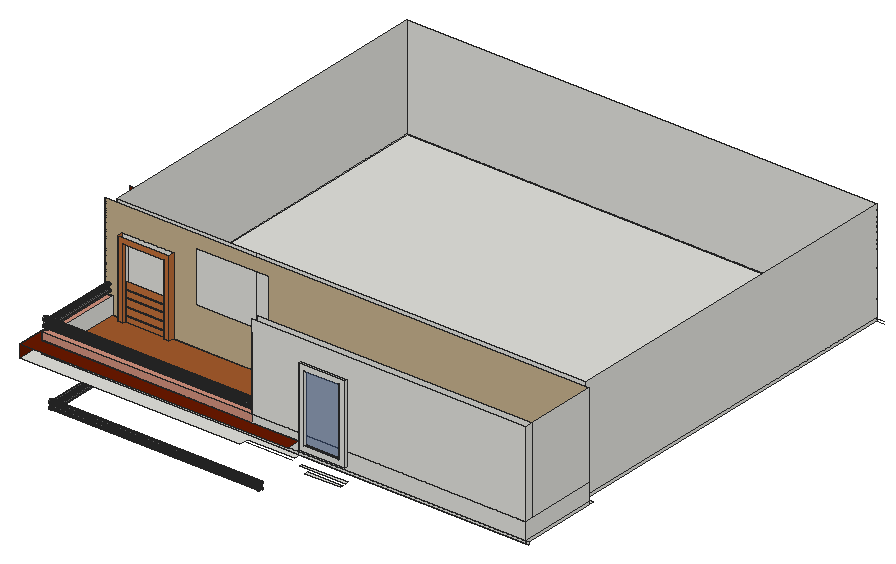
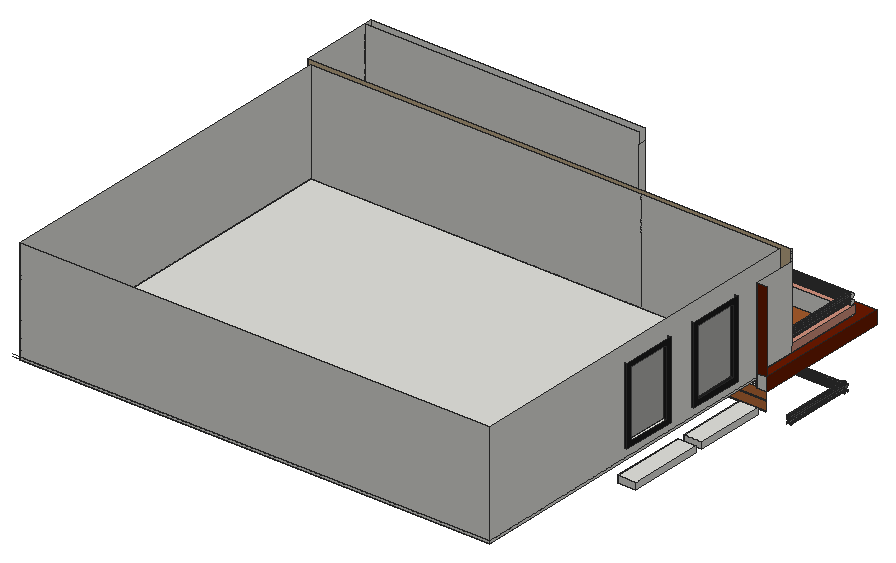
# SketchUp Ruby script. Lengths in inches.
U = 1.inch
M = Sketchup.active_model
def pt(a) = Geom::Point3d.new(a.map { |v| v * U })
def face(e, loops, mat)
  f = e.add_face(loops[0].map { |a| pt(a) })
  loops[1..].each { |l| e.add_face(l.map { |a| pt(a) }).erase! }
  f.material = f.back_material = mat if mat
  f
end
# faces: each face lists its corners as indices into pts; further lists are holes
def faces(e, pts, list, mat = nil) = list.each { |f| face(e, (f[0].is_a?(Array) ? f : [f]).map { |l| l.map { |i| pts[i] } }, mat) }
# xy, xz, yz: faces in a plane at the given z, y or x. An outline is a flat list of corners, or four numbers for a rectangle; further outlines are holes
def ring(l) = l.size == 4 ? [[l[0], l[1]], [l[2], l[1]], [l[2], l[3]], [l[0], l[3]]] : l.each_slice(2).to_a
def flat(e, list, mat, &to3) = list.each { |f| face(e, (f[0].is_a?(Array) ? f : [f]).map { |l| ring(l).map { |u, v| to3.(u, v) } }, mat) }
def xy(e, z, list, mat = nil) = flat(e, list, mat) { |x, y| [x, y, z] }
def xz(e, y, list, mat = nil) = flat(e, list, mat) { |x, z| [x, y, z] }
def yz(e, x, list, mat = nil) = flat(e, list, mat) { |y, z| [x, y, z] }
def lines(e, pts, list) = list.each { |a, b| e.add_line(pt(pts[a]), pt(pts[b])) }
# prism: a flat outline (further loops are holes) pulled along v
def prism(e, loops, v, mat = nil)
  f = face(e, loops, mat); d = Geom::Vector3d.new(v.map { |x| x * U })
  f.pushpull(f.normal.samedirection?(d) ? d.length : -d.length)
end
def box(e, o, s, mat = nil) = prism(e, [[o, [o[0] + s[0], o[1], o[2]], [o[0] + s[0], o[1] + s[1], o[2]], [o[0], o[1] + s[1], o[2]]]], [0, 0, s[2]], mat)
def at(x, y, z, deg = 0) = Geom::Transformation.translation(pt([x, y, z])) * Geom::Transformation.rotation(ORIGIN, Z_AXIS, deg.degrees)
def axes(o, x, y, z) = Geom::Transformation.new([*x, 0, *y, 0, *z, 0, *pt(o).to_a, 1])
def part(name) = M.definitions.add(name)
# library, detail: a bought-in or finely detailed component or shape, given as its bounding box
def library(name, o, s) = part(name).tap { |d| box(d.entities, o, s) }
def detail(e, o, s) = box(e.add_group.entities, o, s)
def put(e, d, t, mat = nil) = e.add_instance(d, t).tap { |i| i.material = mat if mat }
def group(e, t, mat = nil) = e.add_group.tap { |g| g.transformation = t; g.material = mat if mat }.entities
root = M.entities
M.materials.add("[0032_Moccasin]").color = [198, 177, 141]
M.materials.add("[0134_DimGray]").color = [105, 105, 105]
M.materials.add("[Color B02]").color = [209, 145, 125]
M.materials.add("[Color B07]").color = [107, 26, 0]
M.materials.add("[Color M08]").color = [30, 30, 30]
M.materials.add("[Translucent Glass Blue]").color = [61, 91, 145]
M.materials["[Translucent Glass Blue]"].alpha = 0.5
M.materials.add("[Translucent Glass Gray]").color = [128, 128, 128]
M.materials["[Translucent Glass Gray]"].alpha = 0.5
M.materials.add("[Wood Square Tile 01]").color = [164, 91, 44]
M.materials.add("[Wood Veneer 01]").color = [191, 111, 58]
xy(root,210,[[67.4,113.9375,115.4,116.9375],[67.4,116.9375,115.4,119.9375]])
xy(root,216,[[61.4,113.9375,121.4,119.9375]],"[Wood Veneer 01]")
xy(root,222.875,[[152.96,116.9375,192.8,119.9375],[195.8,116.9375,232.65,119.9375]],"[Color M08]")
xy(root,225.875,[[149.96,116.9375,235.65,119.9375]])
xy(root,228.99,[[31.875,209.04,34.875,261.16],[31.875,301.91,34.875,354.04]],"[Color M08]")
xy(root,234.99,[[13.875,196.1,13.875,278.07,34.875,278.07,34.875,267.16,31.875,267.16,31.875,203.04,34.875,203.04,34.875,196.1],[31.875,203.04,34.875,267.16],[13.875,286.99,13.875,375.6,34.875,375.6,34.875,360.04,31.875,360.04,31.875,295.91,34.875,295.91,34.875,286.99],[31.875,295.91,34.875,360.04]])
xy(root,235.15,[[352.1,17.9375,393.78,20.9375]])
xy(root,241.15,[[346.1,17.9375,399.78,20.9375]])
xy(root,242.93,[[13.875,196.1,34.875,278.07],[13.875,286.99,34.875,375.6]])
xy(root,244.83,[[23.625,9.86,23.625,170.67,34.875,170.67,34.875,119.9375,337.625,119.9375,337.625,20.9375,282.125,20.9375,282.125,9.86]])
xy(root,246,[[34.875,26.9375,282.125,37.04],[282.125,26.9375,337.625,37.04],[337.625,26.9375,604.125,44.9375],[34.875,37.04,34.875,119.9375,337.625,119.9375,337.625,44.9375,282.125,44.9375,282.125,37.04],[282.125,37.04,337.625,44.9375],
  [337.625,44.9375,604.125,119.9375],[207.54,119.9375,595.125,125.9375],[595.125,119.9375,603.5625,125.9375],[43.875,125.9375,595.125,552.98]])
xy(root,249,[[34.875,26.9375,34.875,119.9375,43.875,119.9375,43.875,35.9375,595.125,35.9375,595.125,119.9375,604.125,119.9375,604.125,26.9375],[55.4,113.9375,61.4,119.9375],[109.4,113.9375,115.4,119.9375],[61.4,116.9375,109.4,119.9375],[43.875,125.9375,595.125,552.98]])
xy(root,249,[[43.875,35.9375,595.125,35.9375,595.125,119.9375,115.4,119.9375,115.4,113.9375,109.4,113.9375,109.4,116.9375,61.4,116.9375,61.4,113.9375,55.4,113.9375,55.4,119.9375,43.875,119.9375]],"[Wood Square Tile 01]")
xy(root,257.08,[[344.26,17.9375,397.95,20.9375]])
xy(root,260.11,[[23.625,9.86,337.625,9.86,337.625,26.9375,34.875,26.9375,34.875,170.67,23.625,170.67]],"[Color B07]")
xy(root,263.08,[[350.26,17.9375,391.95,20.9375]])
xy(root,266.99,[[31.875,203.04,34.875,267.16],[31.875,301.48,34.875,365.6]],"[Color M08]")
xy(root,268.875,[[282.125,26.9375,604.125,35.9375],[595.125,35.9375,604.125,119.9375]])
xy(root,268.875,[[34.875,26.9375,282.125,26.9375,282.125,35.9375,43.875,35.9375,43.875,119.9375,34.875,119.9375]],"[Color B02]")
xy(root,272.99,[[31.875,307.48,34.875,359.6]])
xy(root,272.99,[[31.875,209.04,34.875,261.16]],"[Color M08]")
xz(root,17.9375,[[[344.26,257.08,397.95,348.9],[350.26,263.08,391.95,342.9]]])
xz(root,20.9375,[[[344.26,257.08,397.95,348.9],[350.26,263.08,391.95,342.9]]])
xz(root,20.9375,[[350.26,263.08,391.95,342.9]],"[Translucent Glass Blue]")
xz(root,26.9375,[[34.875,246,282.125,249],[282.125,246,337.625,249],[337.625,246,604.125,249],[604.125,246,607.125,249],[34.875,249,282.125,260.11],
  [282.125,249,337.625,260.11],[337.625,249,337.625,260.11,282.125,260.11,282.125,268.875,604.125,268.875,604.125,249],[282.125,268.875,604.125,369]])
xz(root,26.9375,[[34.875,260.11,282.125,268.875]],"[Color B02]")
xz(root,29.17,[[39.53,271.5,40.08,271.57,40.59,271.78,41.03,272.12,41.37,272.5625,41.58,273.07,41.66,273.625,41.66,273.63,37.41,273.63,37.41,273.625,37.48,273.07,37.69,272.5625,38.03,272.12,38.47,271.78,38.98,271.57],[37.41,273.63,41.66,273.63,41.58,274.17,41.37,274.6875,41.24,274.86,37.82,274.86,37.69,274.6875,37.48,274.17],[37.82,274.86,41.24,274.86,41.03,275.125,40.59,275.46,40.08,275.68,39.53,275.75,38.98,275.68,38.47,275.46,38.03,275.125]])
xz(root,35.9375,[[43.875,249,282.125,268.875],[282.125,249,595.125,268.875],[282.125,268.875,604.125,369]])
xz(root,113.9375,[[55.4,249,61.4,249,61.4,333,109.4,333,109.4,249,115.4,249,115.4,339,55.4,339]],"[Wood Veneer 01]")
xz(root,116.9375,[[67.4,185.27,115.4,186.19],[67.4,196.84,115.4,197.75],[61.4,255.89,109.4,256.87],[61.4,264.83,109.4,265.81],[61.4,274.08,109.4,275.06],
  [61.4,283.33,109.4,284.31]])
xz(root,116.9375,[[67.4,186.19,115.4,196.84],[67.4,197.75,115.4,210],[61.4,249,109.4,255.89],[61.4,256.87,109.4,264.83],[61.4,265.81,109.4,274.08],
  [61.4,275.06,109.4,283.33],[61.4,284.31,109.4,292.58]],"[Wood Veneer 01]")
xz(root,119.9375,[[34.875,244.83,337.625,246],[34.875,246,43.875,249],[43.875,246,55.4,249],[55.4,246,115.4,249],[115.4,246,207.54,249],
  [207.54,246,595.125,249],[595.125,246,603.4375,249],[603.4375,246,603.5625,249],[603.5625,246,604.125,249],[34.875,249,35.6,268.875],
  [35.6,249,43.875,268.875],[55.4,249,55.4,339,115.4,339,115.4,249,109.4,249,109.4,333,61.4,333,61.4,249],[61.4,249,109.4,333],[595.125,249,603.4375,268.875],[603.4375,249,603.5625,268.875],
  [603.5625,249,604.125,268.875],[34.875,268.875,35.6,369]])
xz(root,119.9375,[[[43.875,249,55.4,249,55.4,339,115.4,339,115.4,249,595.125,249,595.125,268.875,604.125,268.875,604.125,369,35.6,369,35.6,268.875,43.875,268.875],[141.33,293.5,227.02,354.1875],[39.53,271.5,38.98,271.57,38.47,271.78,38.03,272.12,37.69,272.5625,37.48,273.07,37.41,273.625,37.48,274.17,37.69,274.6875,38.03,275.125,38.47,275.46,38.98,275.68,39.53,275.75,40.08,275.68,40.59,275.46,41.03,275.125,41.37,274.6875,41.58,274.17,41.66,273.625,41.58,273.07,41.37,272.5625,41.03,272.12,40.59,271.78,40.08,271.57]]],"[0032_Moccasin]")
xz(root,125.9375,[[43.875,246,207.54,249],[207.54,246,595.125,249],[43.875,249,207.54,369],[207.54,249,595.125,369]])
xz(root,170.67,[[23.625,244.83,34.875,260.11]])
xz(root,170.67,[[23.625,260.11,34.875,355.125]],"[Color B07]")
xz(root,196.1,[[13.875,234.99,34.875,242.93]])
xz(root,203.04,[[31.875,266.99,34.875,357.43]],"[Color M08]")
xz(root,209.04,[[31.875,272.99,34.875,351.43]],"[Color M08]")
xz(root,261.16,[[31.875,272.99,34.875,351.43]],"[Color M08]")
xz(root,267.16,[[31.875,266.99,34.875,357.43]],"[Color M08]")
xz(root,278.07,[[13.875,234.99,34.875,242.93]])
xz(root,286.99,[[13.875,234.99,34.875,242.93]])
xz(root,301.48,[[31.875,266.99,34.875,357.43]],"[Color M08]")
xz(root,307.48,[[31.875,272.99,34.875,351.43]],"[Color M08]")
xz(root,359.6,[[31.875,272.99,34.875,351.43]],"[Color M08]")
xz(root,365.6,[[31.875,266.99,34.875,357.43]],"[Color M08]")
xz(root,375.6,[[13.875,234.99,34.875,242.93]])
xz(root,552.98,[[43.875,246,595.125,249],[43.875,249,595.125,369]])
yz(root,13.875,[[196.1,234.99,278.07,242.93],[286.99,234.99,375.6,242.93]])
yz(root,23.625,[[9.86,244.83,170.67,260.11]],"[Color B07]")
yz(root,31.875,[[[203.04,266.99,267.16,357.43],[209.04,272.99,261.16,351.43]],[[301.48,266.99,365.6,357.43],[307.48,272.99,359.6,351.43]]],"[Color M08]")
yz(root,34.875,[[196.1,234.99,202.6,242.93],[202.6,234.99,278.07,242.93],[286.99,234.99,360.04,242.93],[360.04,234.99,375.6,242.93],[119.9375,244.83,170.67,260.11],
  [26.9375,246,119.9375,249],[26.9375,249,119.9375,260.11],[119.9375,260.11,170.67,355.125],[31.46,271.87,30.85,271.95,30.27,272.1875,29.78,272.5625,29.4,273.06,29.17,273.63,29.09,274.24,29.17,274.86,29.4,275.43,29.78,275.92,30.27,276.3,30.85,276.54,31.46,276.62,32.08,276.54,32.65,276.3,33.14,275.92,33.52,275.43,33.76,274.86,33.84,274.24,33.76,273.63,33.52,273.06,33.14,272.5625,32.65,272.1875,32.08,271.95],[31.46,278.87,30.85,278.95,30.27,279.1875,29.78,279.5625,29.4,280.06,29.17,280.63,29.09,281.24,29.17,281.86,29.4,282.43,29.78,282.92,30.27,283.3,30.85,283.54,31.46,283.62,32.08,283.54,32.65,283.3,33.14,282.92,33.52,282.43,33.76,281.86,33.84,281.24,33.76,280.63,33.52,280.06,33.14,279.5625,32.65,279.1875,32.08,278.95]])
yz(root,34.875,[[40.34,187.58,39.73,187.66,39.15,187.89,38.66,188.27,38.29,188.76,38.05,189.34,37.97,189.95,38.05,190.57,38.29,191.14,38.66,191.63,39.15,192.01,39.73,192.25,40.34,192.33,40.96,192.25,41.53,192.01,42.02,191.63,42.4,191.14,42.64,190.57,42.72,189.95,42.64,189.34,42.4,188.76,42.02,188.27,41.53,187.89,40.96,187.66]],"[0134_DimGray]")
yz(root,34.875,[[26.9375,260.11,119.9375,268.875]],"[Color B02]")
yz(root,34.875,[[209.04,272.99,261.16,351.43],[307.48,272.99,359.6,351.43]],"[Translucent Glass Gray]")
yz(root,43.875,[[125.9375,246,552.98,249],[35.9375,249,119.9375,268.875],[125.9375,249,552.98,369]])
yz(root,55.4,[[113.9375,249,119.9375,339]],"[Wood Veneer 01]")
yz(root,61.4,[[116.9375,249,119.9375,333]])
yz(root,61.4,[[113.9375,249,116.9375,333]],"[Wood Veneer 01]")
yz(root,109.4,[[116.9375,249,119.9375,333]])
yz(root,109.4,[[113.9375,249,116.9375,333]],"[Wood Veneer 01]")
yz(root,115.4,[[113.9375,249,119.9375,339]],"[Wood Veneer 01]")
yz(root,282.125,[[[26.9375,268.875,35.9375,355.125],[31.46,271.87,32.08,271.95,32.65,272.1875,33.14,272.5625,33.52,273.06,33.76,273.63,33.84,274.24,33.76,274.86,33.52,275.43,33.14,275.92,32.65,276.3,32.08,276.54,31.46,276.62,30.85,276.54,30.27,276.3,29.78,275.92,29.4,275.43,29.17,274.86,29.09,274.24,29.17,273.63,29.4,273.06,29.78,272.5625,30.27,272.1875,30.85,271.95],[31.46,278.87,32.08,278.95,32.65,279.1875,33.14,279.5625,33.52,280.06,33.76,280.63,33.84,281.24,33.76,281.86,33.52,282.43,33.14,282.92,32.65,283.3,32.08,283.54,31.46,283.62,30.85,283.54,30.27,283.3,29.78,282.92,29.4,282.43,29.17,281.86,29.09,281.24,29.17,280.63,29.4,280.06,29.78,279.5625,30.27,279.1875,30.85,278.95],[31.46,285.87,32.08,285.95,32.65,286.1875,33.14,286.5625,33.52,287.06,33.76,287.63,33.84,288.24,33.76,288.86,33.52,289.43,33.14,289.92,32.65,290.3,32.08,290.54,31.46,290.62,30.85,290.54,30.27,290.3,29.78,289.92,29.4,289.43,29.17,288.86,29.09,288.24,29.17,287.63,29.4,287.06,29.78,286.5625,30.27,286.1875,30.85,285.95],[31.46,292.87,32.08,292.95,32.65,293.1875,33.14,293.5625,33.52,294.06,33.76,294.63,33.84,295.24,33.76,295.86,33.52,296.43,33.14,296.92,32.65,297.3,32.08,297.54,31.46,297.62,30.85,297.54,30.27,297.3,29.78,296.92,29.4,296.43,29.17,295.86,29.09,295.24,29.17,294.63,29.4,294.06,29.78,293.5625,30.27,293.1875,30.85,292.95],[31.46,299.87,32.08,299.95,32.65,300.1875,33.14,300.5625,33.52,301.06,33.76,301.63,33.84,302.24,33.76,302.86,33.52,303.43,33.14,303.92,32.65,304.3,32.08,304.54,31.46,304.62,30.85,304.54,30.27,304.3,29.78,303.92,29.4,303.43,29.17,302.86,29.09,302.24,29.17,301.63,29.4,301.06,29.78,300.5625,30.27,300.1875,30.85,299.95]]])
yz(root,344.26,[[17.9375,257.08,20.9375,348.9]])
yz(root,350.26,[[17.9375,263.08,20.9375,342.9]])
yz(root,391.95,[[17.9375,263.08,20.9375,342.9]])
yz(root,397.95,[[17.9375,257.08,20.9375,348.9]])
yz(root,595.125,[[119.9375,246,125.9375,249],[125.9375,246,552.98,249],[35.9375,249,110.9375,268.875],[110.9375,249,119.9375,268.875],[125.9375,249,552.98,369]])
yz(root,604.125,[[26.9375,246,119.9375,249],[26.9375,249,119.9375,268.875],[26.9375,268.875,35.9375,369],[35.9375,268.875,119.9375,369]])
p = [[282.125,38.05,182.84],[282.125,37.97,183.45],[34.875,37.97,183.45],[34.875,38.05,182.84],[36.51,38.05,182.84],[41.11,38.05,182.84],
  [36.43,119.9375,183.39],[36.51,119.9375,182.77],[36.51,38.05,182.77],[36.49,38.05,182.94],[36.49,38.05,182.96],[36.43,38.05,183.39],
  [41.1,119.9375,182.77],[41.18,119.9375,183.39],[41.18,38.05,183.39],[41.13,38.05,182.96],[41.125,38.05,182.94],[41.1,38.05,182.77],
  [282.125,42.72,183.45],[282.125,42.64,182.84],[34.875,42.64,182.84],[34.875,42.72,183.45],[36.51,119.9375,184],[36.51,38.05,183.94],
  [36.51,38.05,184],[41.1,119.9375,184],[41.1,38.05,184],[41.11,38.05,183.94],[282.125,38.05,184.07],[41.08,38.05,184.07],
  [36.54,38.05,184.07],[34.875,38.05,184.07],[282.125,42.64,184.07],[34.875,42.64,184.07],[36.75,119.9375,184.57],[36.59,38.05,184.19],
  [36.75,38.05,184.57],[40.87,119.9375,184.57],[40.87,38.05,184.57],[41.02,38.05,184.19],[282.125,38.29,184.64],[34.875,38.29,184.64],
  [282.125,42.4,184.64],[34.875,42.4,184.64],[37.13,119.9375,185.06],[37.13,38.05,185.06],[40.49,119.9375,185.06],[40.49,38.05,185.06],
  [282.125,38.66,185.13],[34.875,38.66,185.13],[282.125,42.02,185.13],[34.875,42.02,185.13],[37.62,119.9375,185.44],[37.62,38.05,185.44],
  [40,119.9375,185.44],[40,38.05,185.44],[282.125,39.15,185.51],[34.875,39.15,185.51],[282.125,41.53,185.51],[34.875,41.53,185.51],
  [38.19,119.9375,185.68],[38.19,38.05,185.68],[39.42,119.9375,185.68],[39.42,38.05,185.68],[282.125,39.73,185.75],[34.875,39.73,185.75],
  [282.125,40.96,185.75],[34.875,40.96,185.75],[38.81,119.9375,185.76],[38.81,38.05,185.76],[282.125,40.34,185.83],[34.875,40.34,185.83],
  [282.125,40.34,187.58],[282.125,39.73,187.66],[34.875,39.73,187.66],[34.875,40.34,187.58],[282.125,40.96,187.66],[34.875,40.96,187.66],
  [282.125,39.15,187.89],[34.875,39.15,187.89],[282.125,41.53,187.89],[34.875,41.53,187.89],[38.19,119.9375,188.03],[38.81,119.9375,187.95],
  [38.81,38.05,187.95],[38.19,38.05,188.03],[39.42,119.9375,188.03],[39.42,38.05,188.03],[282.125,38.66,188.27],[34.875,38.66,188.27],
  [282.125,42.02,188.27],[34.875,42.02,188.27],[37.62,119.9375,188.27],[37.62,38.05,188.27],[40,119.9375,188.27],[40,38.05,188.27],
  [37.13,119.9375,188.64],[37.13,38.05,188.64],[40.49,119.9375,188.64],[40.49,38.05,188.64],[282.125,38.29,188.76],[34.875,38.29,188.76],
  [282.125,42.4,188.76],[34.875,42.4,188.76],[36.75,119.9375,189.14],[37.125,38.05,188.65],[36.75,38.05,189.14],[40.87,119.9375,189.14],
  [40.87,38.05,189.14],[40.49,38.05,188.65],[282.125,38.05,189.34],[40.95,38.05,189.34],[36.67,38.05,189.34],[34.875,38.05,189.34],
  [282.125,42.64,189.34],[34.875,42.64,189.34],[36.51,119.9375,189.71],[36.54,38.05,189.65],[36.51,38.05,189.71],[41.1,119.9375,189.71],
  [41.1,38.05,189.71],[41.08,38.05,189.65],[282.125,37.97,189.95],[34.875,37.97,189.95],[282.125,42.72,189.95],[34.875,42.72,189.95],
  [36.43,119.9375,190.32],[36.51,38.05,189.77],[36.49,38.05,189.88],[36.49,38.05,189.9],[36.43,38.05,190.32],[41.18,119.9375,190.32],
  [41.18,38.05,190.32],[41.13,38.05,189.9],[41.125,38.05,189.88],[41.11,38.05,189.77],[282.125,38.05,190.57],[41.15,38.05,190.57],
  [36.47,38.05,190.57],[34.875,38.05,190.57],[282.125,42.64,190.57],[34.875,42.64,190.57],[36.51,119.9375,190.9375],[36.51,38.05,190.88],
  [36.51,38.05,190.9375],[41.1,119.9375,190.9375],[41.1,38.05,190.9375],[41.11,38.05,190.88],[282.125,38.29,191.14],[34.875,38.29,191.14],
  [282.125,42.4,191.14],[34.875,42.4,191.14],[36.75,119.9375,191.51],[36.54,38.05,191],[36.59,38.05,191.13],[36.75,38.05,191.51],
  [40.87,119.9375,191.51],[40.87,38.05,191.51],[41.02,38.05,191.13],[41.08,38.05,191],[282.125,38.66,191.63],[34.875,38.66,191.63],
  [282.125,42.02,191.63],[34.875,42.02,191.63],[37.13,119.9375,192],[37.13,38.05,192],[40.49,119.9375,192],[40.49,38.05,192],
  [282.125,39.15,192.01],[34.875,39.15,192.01],[282.125,41.53,192.01],[34.875,41.53,192.01],[37.62,119.9375,192.38],[37.62,38.05,192.38],
  [40,119.9375,192.38],[40,38.05,192.38],[282.125,39.73,192.25],[34.875,39.73,192.25],[282.125,40.96,192.25],[34.875,40.96,192.25],
  [282.125,40.34,192.33],[34.875,40.34,192.33],[38.19,119.9375,192.62],[38.19,38.05,192.62],[39.42,119.9375,192.62],[39.42,38.05,192.62],
  [38.81,119.9375,192.7],[38.81,38.05,192.7],[38.98,119.9375,271.57],[39.53,119.9375,271.5],[39.53,29.17,271.5],[38.98,29.17,271.57],
  [40.08,119.9375,271.57],[40.08,29.17,271.57],[38.47,119.9375,271.78],[38.47,29.17,271.78],[40.59,119.9375,271.78],[40.59,29.17,271.78],
  [38.03,119.9375,272.12],[38.03,29.17,272.12],[41.03,119.9375,272.12],[41.03,29.17,272.12],[282.125,30.85,271.95],[282.125,30.27,272.1875],
  [34.875,30.27,272.1875],[34.875,30.85,271.95],[282.125,31.46,271.87],[34.875,31.46,271.87],[282.125,32.08,271.95],[34.875,32.08,271.95],
  [282.125,32.65,272.1875],[34.875,32.65,272.1875],[37.69,119.9375,272.5625],[37.69,29.17,272.5625],[41.37,119.9375,272.5625],[41.37,29.17,272.5625],
  [282.125,29.78,272.5625],[34.875,29.78,272.5625],[282.125,33.14,272.5625],[34.875,33.14,272.5625],[37.48,119.9375,273.07],[37.48,29.17,273.07],
  [41.58,119.9375,273.07],[41.58,29.17,273.07],[282.125,29.4,273.06],[34.875,29.4,273.06],[282.125,33.52,273.06],[34.875,33.52,273.06],
  [282.125,29.17,273.63],[41.66,29.17,273.63],[37.41,29.17,273.63],[34.875,29.17,273.63],[37.41,119.9375,273.625],[37.41,29.17,273.625],
  [41.66,119.9375,273.625],[41.66,29.17,273.625],[282.125,33.76,273.63],[34.875,33.76,273.63],[282.125,29.09,274.24],[34.875,29.09,274.24],
  [37.48,119.9375,274.17],[37.48,29.17,274.17],[41.58,119.9375,274.17],[41.58,29.17,274.17],[282.125,33.84,274.24],[34.875,33.84,274.24],
  [282.125,29.17,274.86],[41.24,29.17,274.86],[37.82,29.17,274.86],[34.875,29.17,274.86],[37.69,119.9375,274.6875],[37.69,29.17,274.6875],
  [41.37,119.9375,274.6875],[41.37,29.17,274.6875],[282.125,33.76,274.86],[34.875,33.76,274.86],[38.03,119.9375,275.125],[38.03,29.17,275.125],
  [41.03,119.9375,275.125],[41.03,29.17,275.125],[282.125,29.4,275.43],[34.875,29.4,275.43],[282.125,33.52,275.43],[34.875,33.52,275.43],
  [38.47,119.9375,275.46],[38.47,29.17,275.46],[40.59,119.9375,275.46],[40.59,29.17,275.46],[282.125,29.78,275.92],[34.875,29.78,275.92],
  [282.125,33.14,275.92],[34.875,33.14,275.92],[38.98,119.9375,275.68],[38.98,29.17,275.68],[40.08,119.9375,275.68],[40.08,29.17,275.68],
  [39.53,119.9375,275.75],[39.53,29.17,275.75],[282.125,30.27,276.3],[34.875,30.27,276.3],[282.125,32.65,276.3],[34.875,32.65,276.3],
  [282.125,30.85,276.54],[34.875,30.85,276.54],[282.125,32.08,276.54],[34.875,32.08,276.54],[282.125,31.46,276.62],[34.875,31.46,276.62],
  [38.98,119.9375,278.38],[39.53,119.9375,278.3125],[39.53,29.17,278.3125],[38.98,29.17,278.38],[40.08,119.9375,278.38],[40.08,29.17,278.38],
  [38.47,119.9375,278.6],[38.47,29.17,278.6],[40.59,119.9375,278.6],[40.59,29.17,278.6],[38.03,119.9375,278.93],[38.03,29.17,278.93],
  [41.03,119.9375,278.93],[41.03,29.17,278.93],[37.69,119.9375,279.375],[37.69,29.17,279.375],[41.37,119.9375,279.375],[41.37,29.17,279.375],
  [282.125,30.85,278.95],[282.125,30.27,279.1875],[34.875,30.27,279.1875],[34.875,30.85,278.95],[282.125,31.46,278.87],[34.875,31.46,278.87],
  [282.125,32.08,278.95],[34.875,32.08,278.95],[282.125,32.65,279.1875],[34.875,32.65,279.1875],[282.125,29.78,279.5625],[34.875,29.78,279.5625],
  [282.125,33.14,279.5625],[34.875,33.14,279.5625],[37.48,119.9375,279.89],[37.48,29.17,279.89],[41.58,119.9375,279.89],[41.58,29.17,279.89],
  [282.125,29.4,280.06],[34.875,29.4,280.06],[282.125,33.52,280.06],[34.875,33.52,280.06],[37.41,119.9375,280.4375],[37.41,29.17,280.4375],
  [41.66,119.9375,280.4375],[41.66,29.17,280.4375],[282.125,29.17,280.63],[41.63,29.17,280.63],[37.43,29.17,280.63],[34.875,29.17,280.63],
  [282.125,33.76,280.63],[34.875,33.76,280.63],[37.48,119.9375,280.99],[37.41,29.17,280.44],[37.48,29.17,280.99],[41.58,119.9375,280.99],
  [41.58,29.17,280.99],[41.66,29.17,280.44],[282.125,29.09,281.24],[34.875,29.09,281.24],[282.125,33.84,281.24],[34.875,33.84,281.24],
  [37.69,119.9375,281.5],[37.69,29.17,281.5],[41.37,119.9375,281.5],[41.37,29.17,281.5],[282.125,29.17,281.86],[41.1,29.17,281.86],
  [37.97,29.17,281.86],[34.875,29.17,281.86],[282.125,33.76,281.86],[34.875,33.76,281.86],[38.03,119.9375,281.9375],[37.82,29.17,281.67],
  [38.03,29.17,281.9375],[41.03,119.9375,281.9375],[41.03,29.17,281.9375],[41.24,29.17,281.67],[282.125,29.4,282.43],[34.875,29.4,282.43],
  [38.47,119.9375,282.28],[38.47,29.17,282.28],[40.59,119.9375,282.28],[40.59,29.17,282.28],[282.125,33.52,282.43],[34.875,33.52,282.43],
  [38.98,119.9375,282.49],[38.98,29.17,282.49],[40.08,119.9375,282.49],[40.08,29.17,282.49],[282.125,29.78,282.92],[34.875,29.78,282.92],
  [282.125,33.14,282.92],[34.875,33.14,282.92],[39.53,119.9375,282.5625],[39.53,29.17,282.5625],[282.125,30.27,283.3],[34.875,30.27,283.3],
  [282.125,32.65,283.3],[34.875,32.65,283.3],[282.125,30.85,283.54],[34.875,30.85,283.54],[282.125,32.08,283.54],[34.875,32.08,283.54],
  [282.125,31.46,283.62],[34.875,31.46,283.62],[595.125,552.98,246],[604.125,552.98,246],[595.125,552.98,249],[604.125,552.98,249],
  [603.5625,125.9375,246],[604.125,125.9375,246],[282.125,16.42,244.83],[337.625,16.42,244.83]]
faces(root,p,[[0,1,2,3,4,5],[6,7,8,4,9,10,11],[12,13,14,15,16,5,17],[18,19,20,21],[22,6,11,23,24],[13,25,26,27,14],[1,28,29,30,31,2],[32,18,21,33],
  [34,22,24,30,35,36],[25,37,38,39,29,26],[28,40,41,31,30,29],[42,32,33,43],[44,34,36,45],[37,46,47,38],[40,48,49,41],[50,42,43,51],
  [52,44,45,53],[46,54,55,47],[48,56,57,49],[58,50,51,59],[60,52,53,61],[54,62,63,55],[56,64,65,57],[66,58,59,67],
  [68,60,61,69],[62,68,69,63],[64,70,71,65],[70,66,67,71],[72,73,74,75],[76,72,75,77],[73,78,79,74],[80,76,77,81],
  [82,83,84,85],[83,86,87,84],[78,88,89,79],[90,80,81,91],[92,82,85,93],[86,94,95,87],[96,92,93,97],[94,98,99,95],
  [88,100,101,89],[102,90,91,103],[104,96,97,105,106],[98,107,108,109,99],[100,110,111,112,113,101],[114,102,103,115],[116,104,106,112,117,118],[107,119,120,121,111,108],
  [110,122,123,113,112,111],[124,114,115,125],[126,116,118,127,128,129,130],[119,131,132,133,134,135,120],[122,136,137,138,139,123],[140,124,125,141],[142,126,130,138,143,144],[131,145,146,147,137,132],
  [136,148,149,139,138,137],[150,140,141,151],[152,142,144,153,154,155],[145,156,157,158,159,146],[148,160,161,149],[162,150,151,163],[164,152,155,165],[156,166,167,157],
  [160,168,169,161],[170,162,163,171],[172,164,165,173],[166,174,175,167],[168,176,177,169],[178,170,171,179],[176,180,181,177],[180,178,179,181],
  [182,172,173,183],[174,184,185,175],[186,182,183,187],[184,186,187,185],[188,189,190,191],[189,192,193,190],[194,188,191,195],[192,196,197,193],
  [198,194,195,199],[196,200,201,197],[202,203,204,205],[206,202,205,207],[208,206,207,209],[210,208,209,211],[212,198,199,213],[200,214,215,201],
  [203,216,217,204],[218,210,211,219],[220,212,213,221],[214,222,223,215],[216,224,225,217],[226,218,219,227],[224,228,229,230,231,225],[232,220,221,233],
  [222,234,235,223],[236,226,227,237],[228,238,239,231,230,229],[240,232,233,230,241],[234,242,243,229,235],[244,236,237,245],[238,246,247,248,249,239],[250,240,241,251],
  [242,252,253,243],[254,244,245,255],[256,250,251,248,257],[252,258,259,247,253],[246,260,261,249,248,247],[262,254,255,263],[264,256,257,265],[258,266,267,259],
  [260,268,269,261],[270,262,263,271],[272,264,265,273],[266,274,275,267],[276,272,273,277],[274,276,277,275],[268,278,279,269],[280,270,271,281],
  [278,282,283,279],[284,280,281,285],[282,286,287,283],[286,284,285,287],[288,289,290,291],[289,292,293,290],[294,288,291,295],[292,296,297,293],
  [298,294,295,299],[296,300,301,297],[302,298,299,303],[300,304,305,301],[306,307,308,309],[310,306,309,311],[312,310,311,313],[314,312,313,315],
  [307,316,317,308],[318,314,315,319],[320,302,303,321],[304,322,323,305],[316,324,325,317],[326,318,319,327],[328,320,321,329],[322,330,331,323],
  [324,332,333,334,335,325],[336,326,327,337],[338,328,329,339,334,340],[330,341,342,333,343,331],[332,344,345,335,334,333],[346,336,337,347],[348,338,340,349],[341,350,351,342],
  [344,352,353,354,355,345],[356,346,347,357],[358,348,349,359,354,360],[350,361,362,353,363,351],[352,364,365,355,354,353],[366,358,360,367],[361,368,369,362],[370,356,357,371],
  [372,366,367,373],[368,374,375,369],[364,376,377,365],[378,370,371,379],[380,372,373,381],[374,380,381,375],[376,382,383,377],[384,378,379,385],
  [382,386,387,383],[388,384,385,389],[386,390,391,387],[390,388,389,391]],"[0134_DimGray]")
lines(root,p,[[392,393],[394,395],[396,397],[398,399]])
